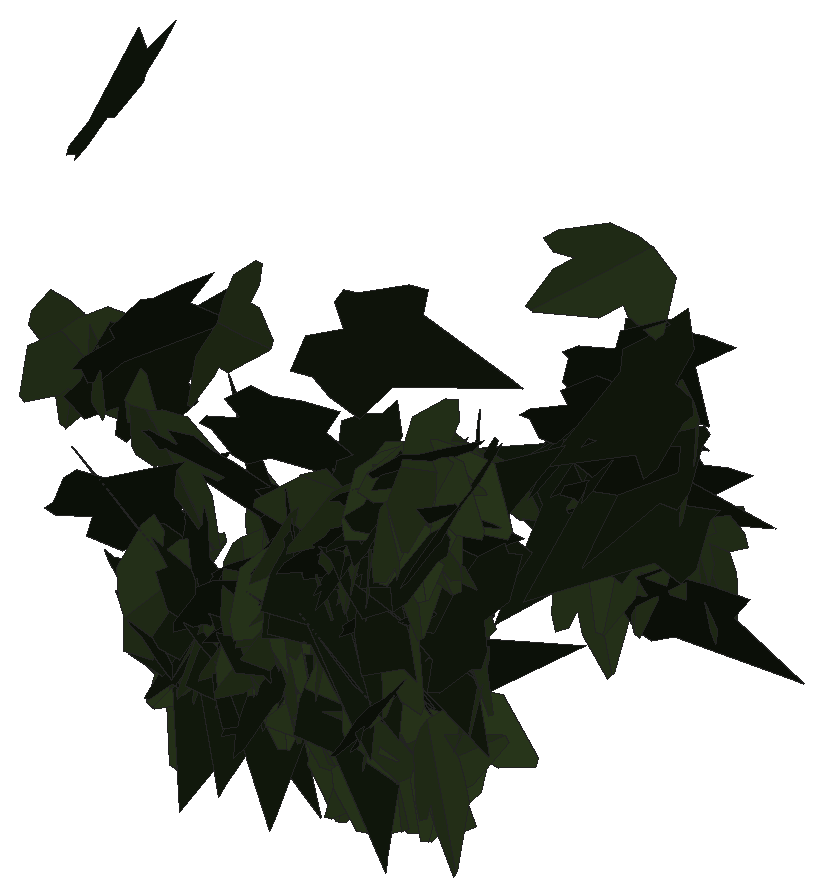
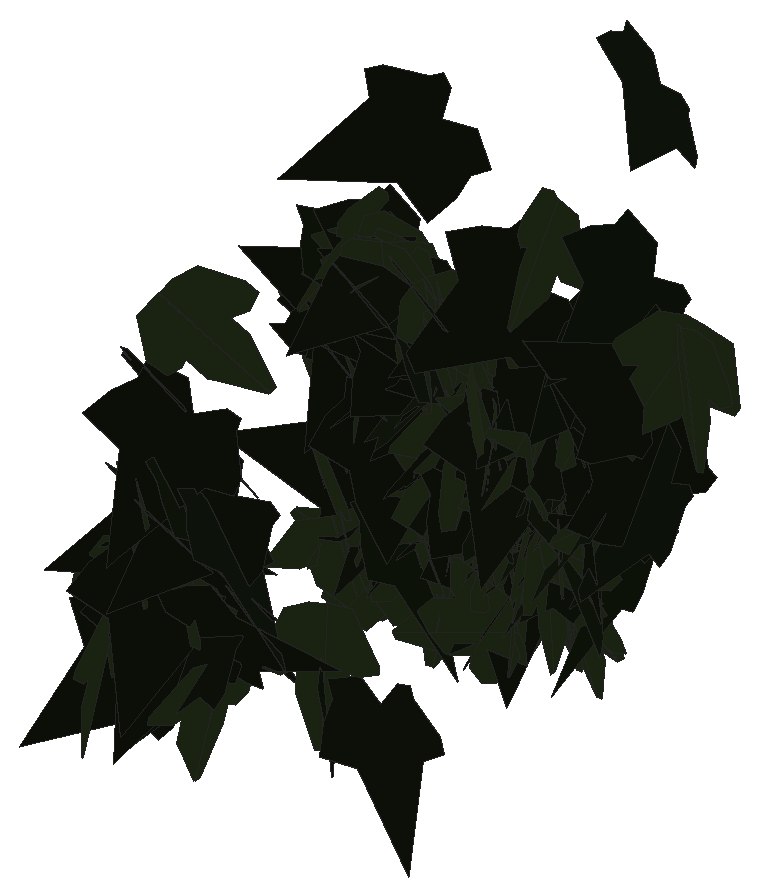
# SketchUp Ruby script. Lengths in inches.
U = 1.inch
M = Sketchup.active_model
def pt(a) = Geom::Point3d.new(a.map { |v| v * U })
def face(e, loops, mat)
  f = e.add_face(loops[0].map { |a| pt(a) })
  loops[1..].each { |l| e.add_face(l.map { |a| pt(a) }).erase! }
  f.material = f.back_material = mat if mat
  f
end
# faces: each face lists its corners as indices into pts; further lists are holes
def faces(e, pts, list, mat = nil) = list.each { |f| face(e, (f[0].is_a?(Array) ? f : [f]).map { |l| l.map { |i| pts[i] } }, mat) }
# xy, xz, yz: faces in a plane at the given z, y or x. An outline is a flat list of corners, or four numbers for a rectangle; further outlines are holes
def ring(l) = l.size == 4 ? [[l[0], l[1]], [l[2], l[1]], [l[2], l[3]], [l[0], l[3]]] : l.each_slice(2).to_a
def flat(e, list, mat, &to3) = list.each { |f| face(e, (f[0].is_a?(Array) ? f : [f]).map { |l| ring(l).map { |u, v| to3.(u, v) } }, mat) }
def xy(e, z, list, mat = nil) = flat(e, list, mat) { |x, y| [x, y, z] }
def xz(e, y, list, mat = nil) = flat(e, list, mat) { |x, z| [x, y, z] }
def yz(e, x, list, mat = nil) = flat(e, list, mat) { |y, z| [x, y, z] }
def lines(e, pts, list) = list.each { |a, b| e.add_line(pt(pts[a]), pt(pts[b])) }
# prism: a flat outline (further loops are holes) pulled along v
def prism(e, loops, v, mat = nil)
  f = face(e, loops, mat); d = Geom::Vector3d.new(v.map { |x| x * U })
  f.pushpull(f.normal.samedirection?(d) ? d.length : -d.length)
end
def box(e, o, s, mat = nil) = prism(e, [[o, [o[0] + s[0], o[1], o[2]], [o[0] + s[0], o[1] + s[1], o[2]], [o[0], o[1] + s[1], o[2]]]], [0, 0, s[2]], mat)
def at(x, y, z, deg = 0) = Geom::Transformation.translation(pt([x, y, z])) * Geom::Transformation.rotation(ORIGIN, Z_AXIS, deg.degrees)
def axes(o, x, y, z) = Geom::Transformation.new([*x, 0, *y, 0, *z, 0, *pt(o).to_a, 1])
def part(name) = M.definitions.add(name)
# library, detail: a bought-in or finely detailed component or shape, given as its bounding box
def library(name, o, s) = part(name).tap { |d| box(d.entities, o, s) }
def detail(e, o, s) = box(e.add_group.entities, o, s)
def put(e, d, t, mat = nil) = e.add_instance(d, t).tap { |i| i.material = mat if mat }
def group(e, t, mat = nil) = e.add_group.tap { |g| g.transformation = t; g.material = mat if mat }.entities
root = M.entities
M.materials.add("efeu1").color = [18, 25, 13]
M.materials.add("efeu2").color = [43, 57, 29]
c1 = part("ivyleaf_9")
p = [[1.54,2.16,1.25],[1.36,2.04,1.19],[-0.21,0.99,0.68],[-0.71,1.11,0.82],[-0.85,0.86,0.67],[-0.8,0.17,0.21],
  [-0.9,-0.01,0.1],[-0.67,-0.16,-0.02],[-0.08,-0.08,-0.05],[-0.03,-0.6,-0.4],[0.65,-0.88,-0.66],[0.83,-0.6,-0.49],
  [1.29,-0.42,-0.43],[1.8125,-0.07,-0.26],[1.21,0.44,0.15]]
faces(c1.entities,p,[[0,1,2,3,4,5,6,7,8,9,10,11,12,13,14]],"efeu1")
c2 = part("ivyleaf_10")
p = [[0,0.5,-0.03],[-0.0625,2.02,-0.43],[-0.19,2.01,-0.46],[-0.54,1.05,-0.29],[-0.52,0.625,-0.18],[-0.83,0.76,-0.28],
  [-1.16,0.64,-0.33],[-1.15,0.33,-0.24],[-0.77,-0.39,0.02],[-0.3,-0.51,0.16],[0.04,-0.48,0.23],[-0.02,2.01,-0.4375],
  [-0.06,2.01,-0.43],[0.04,-0.49,0.23],[0.67,-0.49,0.14],[1.38,0.36,-0.2],[1.375,0.51,-0.24],[0.81,0.65,-0.19],
  [0.62,0.59,-0.15],[0.6,1.09,-0.28],[0.5,1.23,-0.31]]
faces(c2.entities,p,[[0,1,2,3,4,5,6,7,8,9,10],[11,12,0,13,14,15,16,17,18,19,20]],"efeu2")
put(root,c1,axes([30.3,224.34,224.28],[0.36199,0.32235,-0.1227],[0.08167,0.09271,0.48449],[0.3351,-0.37081,0.01446]))
put(root,c2,axes([32.81,224.46,225.28],[-0.03829,-0.49672,-0.04244],[-0.01517,0.0437,-0.49786],[0.4983,-0.03683,-0.01841]))
put(root,c2,axes([30.12,224.32,225.76],[-0.34431,-0.24602,-0.26632],[0.22559,0.14214,-0.42297],[0.28383,-0.41142,0.01312]))
put(root,c1,axes([31.24,224.25,225.24],[0.49836,0.04008,-0.00536],[-0.00887,0.04369,-0.49801],[-0.03945,0.49647,0.04426]))
put(root,c1,axes([32.05,224.4,223.45],[-0.3806,0.32371,0.01877],[-0.01525,0.01104,-0.49965],[-0.3239,-0.3809,0.00148]))
put(root,c1,axes([31.45,224.68,223.42],[-0.37688,-0.29912,-0.13597],[0.14267,0.03742,-0.47775],[0.29598,-0.39891,0.05715]))
put(root,c2,axes([30.91,224.42,225.18],[-0.45546,0.1255,-0.16373],[0.1574,-0.0451,-0.47243],[-0.13335,-0.48189,0.00157]))
put(root,c2,axes([30,224.39,225.77],[0.44133,-0.1976,-0.12722],[-0.05473,0.17682,-0.46448],[0.22855,0.4239,0.13444]))
put(root,c2,axes([32.14,224.55,224.76],[0.14337,-0.47824,0.02696],[0.00611,-0.02632,-0.49927],[0.47896,0.14349,-0.0017]))
put(root,c2,axes([31.86,224.5625,223.79],[-0.30924,0.2654,-0.28972],[0.18417,-0.22777,-0.40522],[-0.34707,-0.35733,0.04311]))
put(root,c1,axes([32.98,224.1875,226.95],[0.03794,0.09374,-0.48967],[0.18461,0.45354,0.10112],[0.46312,-0.18846,-0.0002]))
put(root,c2,axes([33.05,224.51,224.05],[0.47753,-0.11742,-0.09043],[-0.08349,0.03892,-0.49144],[0.12245,0.48446,0.01756]))
put(root,c1,axes([33,224.52,225.51],[-0.45583,0.20506,-0.0131],[0.00986,-0.01002,-0.4998],[-0.20524,-0.45591,0.00509]))
put(root,c2,axes([31.29,224.49,223.57],[0.20122,-0.45427,-0.05611],[0.03844,0.07785,-0.4924],[0.4561,0.19385,0.06626]))
put(root,c2,axes([33.43,224.54,225.62],[0.4997,0.01296,-0.01164],[-0.01166,0.00038,-0.49986],[-0.01295,0.49983,0.00068]))
put(root,c1,axes([31.86,224.26,224.24],[0.16464,0.46751,-0.06579],[-0.01741,-0.06361,-0.49563],[-0.47179,0.16549,-0.00466]))
put(root,c2,axes([33.6,224.57,225.69],[0.3653,0.27747,-0.1989],[-0.17977,-0.09131,-0.45754],[-0.29024,0.4058,0.03305]))
put(root,c2,axes([33.35,224.46,225.56],[-0.44466,-0.17136,-0.15137],[0.16363,-0.00729,-0.47241],[0.1597,-0.46966,0.06256]))
put(root,c2,axes([32.6,224.5,225.06],[-0.44918,-0.20095,0.08865],[-0.0734,-0.05288,-0.49175],[0.20701,-0.45478,0.01801]))
put(root,c1,axes([30.7,224.1,226.14],[0.21613,0.35999,0.27146],[0.11023,0.24971,-0.41892],[-0.43719,0.24093,0.02858]))
put(root,c2,axes([33.17,224.45,225.08],[-0.49791,-0.04403,0.01222],[-0.0124,0.00159,-0.49984],[0.04398,-0.49805,-0.00267]))
put(root,c1,axes([30.5625,224.12,228.125],[0.0463,0.33401,0.36918],[-0.07892,0.37101,-0.32576],[-0.49156,-0.02811,0.08707]))
put(root,c1,axes([31.86,224.27,225.72],[0.45476,0.1337,0.15911],[0.153,0.04367,-0.47401],[-0.14065,0.47981,-0.00119]))
put(root,c1,axes([33.55,224.52,225.26],[-0.42667,0.25335,0.06137],[-0.07135,-0.00027,-0.49488],[-0.25072,-0.43106,0.03639]))
put(root,c2,axes([30.88,224.13,223.8],[0.02789,0.03793,-0.49778],[0.13057,0.48065,0.04394],[0.48184,-0.13244,0.0169]))
put(root,c2,axes([32.77,224.5,224.96],[0.31589,-0.354,-0.15778],[-0.09579,0.12593,-0.47431],[0.37555,0.32988,0.01174]))
put(root,c1,axes([32.53,224.69,224.5],[-0.01567,-0.49138,-0.09112],[-0.00161,0.09121,-0.49161],[0.49975,-0.01511,-0.00444]))
put(root,c1,axes([31.61,224.73,223.64],[-0.34414,-0.32276,-0.16552],[0.13104,0.10213,-0.47159],[0.33823,-0.36796,0.0143]))
put(root,c2,axes([33.3,224.49,225.59],[0.31849,0.37839,0.07338],[0.04371,0.05912,-0.49456],[-0.38296,0.32144,0.00458]))
put(root,c2,axes([31.68,224.52,224.18],[-0.04676,0.49437,-0.05844],[0.0001,-0.05868,-0.49654],[-0.49781,-0.04645,0.00539]))
put(root,c2,axes([32.6,224.48,224.96],[0.36442,-0.23007,-0.25351],[-0.18601,0.17777,-0.42872],[0.2874,0.40678,0.04398]))
put(root,c2,axes([33.35,224.51,225.26],[0.04972,0.49715,-0.01931],[-0.02432,-0.01696,-0.49912],[-0.49693,0.05057,0.02249]))
put(root,c2,axes([32.1,224.49,224.29],[0.25045,0.42741,0.06776],[0.03524,0.05789,-0.49539],[-0.43132,0.25291,-0.00112]))
put(root,c2,axes([31.39,224.61,223.27],[0.44892,-0.21518,-0.0466],[-0.04186,0.02049,-0.49782],[0.21615,0.45086,0.00038]))
put(root,c2,axes([31.78,224.46,223.94],[-0.34665,-0.25569,-0.25388],[0.24054,0.09808,-0.42722],[0.26828,-0.41833,0.05501]))
put(root,c1,axes([31.35,224.41,224.21],[0.10228,0.00438,-0.48941],[-0.48941,0.00532,-0.10223],[0.00431,0.49995,0.00537]))
put(root,c1,axes([31.7,224.8,223.33],[-0.02516,-0.4992,-0.0128],[0.00071,0.01278,-0.49984],[0.49937,-0.02516,0.00007]))
put(root,c1,axes([32.83,224.54,224.97],[-0.34487,0.35707,-0.05969],[0.03523,-0.04895,-0.49635],[-0.36031,-0.34656,0.0086]))
put(root,c2,axes([31.58,224.32,226.47],[-0.02562,-0.32422,-0.37977],[0.02402,0.37902,-0.32521],[0.49876,-0.03491,-0.00384]))
put(root,c1,axes([32.39,224.73,224.25],[0.09337,-0.48739,-0.0611],[-0.00082,0.06204,-0.49614],[0.4912,0.09275,0.01078]))
put(root,c1,axes([32.88,224.51,224.92],[-0.0032,0.44388,-0.23014],[-0.06967,-0.22829,-0.43935],[-0.49511,0.02925,0.06332]))
put(root,c1,axes([32.59,224.64,224.52],[-0.14359,-0.35991,-0.31598],[0.18205,0.2641,-0.38355],[0.44299,-0.2252,0.0552]))
put(root,c1,axes([32.6,224.78,223.25],[0.10058,-0.48957,0.01421],[0.00681,-0.01311,-0.49978],[0.48973,0.10073,0.00403]))
put(root,c1,axes([32.97,224.39,223.22],[0.05274,0.49685,0.01892],[-0.00193,-0.01882,0.49964],[0.49721,-0.05277,-0.00007]))
put(root,c1,axes([32.4,224.57,223.78],[0.43778,-0.23928,0.03305],[0.02907,-0.01573,-0.49891],[0.2398,0.43875,0.00014]))
put(root,c2,axes([32.85,224.89,222.76],[-0.17744,-0.18713,-0.42836],[-0.27686,-0.3271,0.25758],[-0.37664,0.32861,0.01246]))
put(root,c2,axes([32,224.6,223.6],[-0.09185,-0.48876,-0.05174],[0.00474,0.05176,-0.49729],[0.49147,-0.09185,-0.00488]))
put(root,c1,axes([30.59,224.38,223.61],[0.40946,-0.07041,-0.27819],[-0.24524,0.16583,-0.40294],[0.14901,0.46641,0.10126]))
put(root,c1,axes([33.86,224.43,225.54],[-0.22701,0.43879,0.07699],[-0.02501,0.07371,-0.4939],[-0.44479,-0.2281,-0.01152]))
put(root,c2,axes([31.67,224.67,223.65],[0.03199,-0.49883,-0.01207],[0.00001,0.0121,-0.49985],[0.49898,0.03198,0.00078]))
put(root,c1,axes([31.32,224.33,223.51],[-0.11731,0.40517,0.26847],[-0.11976,0.24357,-0.41992],[-0.47106,-0.16282,0.0399]))
put(root,c1,axes([30.17,224.51,224.46],[0.47288,-0.11244,-0.11724],[-0.10971,0.04507,-0.48573],[0.1198,0.4851,0.01796]))
put(root,c1,axes([31.51,224.65,223.65],[0.34569,-0.3611,-0.01008],[0.05427,0.06571,-0.49268],[0.35714,0.33954,0.08462]))
put(root,c2,axes([32.14,224.6,224.41],[-0.36525,0.33105,-0.08364],[0.05588,-0.06287,-0.49287],[-0.33685,-0.36939,0.00893]))
put(root,c2,axes([31.04,224.7,223.12],[0.47205,-0.16472,-0.00586],[-0.0047,0.00431,-0.49996],[0.16476,0.47207,0.00252]))
put(root,c1,axes([31.02,224.375,224.01],[0.38554,-0.03908,-0.31596],[-0.26335,0.23969,-0.35099],[0.1789,0.43706,0.16424]))
put(root,c2,axes([31.88,224.61,223.6875],[0.23827,0.43931,0.01538],[0.00833,0.01297,-0.49976],[-0.4395,0.23841,-0.00114]))
put(root,c1,axes([32.04,224.625,223.93],[-0.06961,0.42991,-0.24563],[-0.07281,-0.25424,-0.42434],[-0.48975,-0.02331,0.098]))
put(root,c2,axes([32.125,224.7,224.03],[-0.05275,-0.49721,-0.00051],[-0.0003,0.00054,-0.5],[0.49721,-0.05275,-0.00035]))
put(root,c2,axes([33.51,224.625,223.12],[-0.09083,0.49094,-0.02695],[0.00194,-0.02705,-0.49926],[-0.49168,-0.0908,0.00301]))
put(root,c2,axes([32.33,224.51,224.02],[0.27172,-0.20687,-0.3652],[-0.23163,0.2889,-0.33599],[0.35002,0.35177,0.06116]))
put(root,c2,axes([32.45,224.66,224.61],[-0.48803,0.09488,0.05317],[-0.06693,-0.0693,-0.49063],[-0.08573,-0.486,0.08034]))
put(root,c2,axes([33.5,224.38,225.82],[0.01346,-0.24934,-0.43319],[0.16225,0.41206,-0.23213],[0.47275,-0.13432,0.09201]))
put(root,c2,axes([32.57,224.78,223.12],[-0.35216,-0.34422,0.08658],[0.01571,-0.13696,-0.48062],[0.3546,-0.33579,0.10727]))
put(root,c1,axes([34.01,224.54,224.55],[-0.29796,0.27833,0.28941],[-0.21545,0.19329,-0.4077],[-0.33883,-0.36766,0.00475]))
put(root,c1,axes([33.15,224.7,224.42],[0.1747,-0.42786,-0.19084],[-0.00516,0.20191,-0.45739],[0.46846,0.16178,0.06613]))
put(root,c1,axes([33.375,224.44,225.06],[0.00619,0.00028,0.49996],[0.4729,0.16226,-0.00594],[-0.16225,0.47294,0.00175]))
put(root,c1,axes([33.19,224.3125,225.61],[0.32859,0.3029,0.22423],[0.09206,0.22398,-0.43745],[-0.36545,0.32877,0.09143]))
put(root,c2,axes([31.24,224.77,223.4],[0.42305,-0.0053,-0.26645],[-0.2665,-0.0045,-0.42304],[0.00209,0.49995,-0.00663]))
put(root,c1,axes([33.35,224.46,225.15],[0.37723,0.32662,-0.0319],[-0.01898,-0.02682,-0.49892],[-0.32763,0.37762,-0.00784]))
put(root,c2,axes([32.41,224.65,223.02],[-0.49881,0.03189,-0.01316],[0.01301,-0.00282,-0.49982],[-0.03195,-0.49897,0.00199]))
put(root,c2,axes([32.8,224.63,224.86],[0.31205,-0.36083,-0.14976],[0.015,0.20259,-0.45687],[0.39039,0.28064,0.13726]))
put(root,c1,axes([31.48,224.74,223.28],[0.27046,-0.39556,-0.14278],[-0.08257,0.1165,-0.47918],[0.41235,0.28277,-0.0023]))
put(root,c1,axes([31.92,224.6,224.4],[0.09363,-0.17736,0.45801],[-0.1806,0.42116,0.20001],[-0.45674,-0.20289,0.01481]))
put(root,c1,axes([31.25,224.55,223.58],[0.49811,0.04244,-0.00934],[-0.01129,0.02258,-0.49936],[-0.04196,0.49768,0.02345]))
put(root,c1,axes([31.83,224.64,223.93],[0.44406,-0.2255,0.04427],[0.10052,0.10399,-0.47863],[0.20665,0.43398,0.13769]))
put(root,c2,axes([32.34,224.62,224.43],[0.13376,0.47382,0.08717],[-0.0554,0.10499,-0.4857],[-0.47858,0.12028,0.08058]))
put(root,c2,axes([32.66,224.77,223.54],[0.23852,0.43288,-0.07566],[-0.04254,-0.06294,-0.4942],[-0.43738,0.24219,0.00681]))
put(root,c1,axes([32.67,224.69,224.67],[0.37045,-0.32576,-0.08156],[0.02413,0.14694,-0.47731],[0.33494,0.3497,0.12459]))
put(root,c2,axes([31.26,224.75,223.48],[0.0405,-0.49155,-0.0821],[0.01724,0.0837,-0.49264],[0.49806,0.03707,0.02373]))
put(root,c2,axes([31.53,224.77,223.35],[-0.18545,-0.45836,-0.07426],[0.04571,0.06156,-0.49409],[0.46208,-0.19005,0.01907]))
put(root,c1,axes([31.83,224.49,224.38],[0.14163,0.47564,0.06085],[-0.0301,0.07214,-0.49385],[-0.47857,0.13623,0.04907]))
put(root,c2,axes([32.14,224.6,224.06],[-0.33084,0.26799,0.26216],[-0.2152,0.15054,-0.42547],[-0.30698,-0.39436,0.01573]))
put(root,c2,axes([31.84,224.67,224.06],[0.41877,0.01933,0.2725],[-0.27118,0.08965,0.41039],[-0.033,-0.49152,0.08557]))
put(root,c2,axes([33.01,224.69,222.49],[0.06564,0.48943,-0.07844],[0.01477,0.07716,0.49379],[0.49545,-0.06714,-0.00433]))
put(root,c2,axes([32.61,224.87,223.21],[0.3514,-0.35349,-0.03959],[-0.02626,0.02972,-0.49842],[0.35472,0.35237,0.00232]))
put(root,c2,axes([33.07,224.6875,222.62],[-0.22767,-0.19052,0.40233],[0.30842,0.25836,0.29687],[-0.32101,0.38335,-0.00012]))
put(root,c1,axes([31.68,224.68,223.49],[0.29649,0.33224,-0.2274],[-0.15624,-0.16532,-0.44526],[-0.37106,0.33509,0.00578]))
put(root,c1,axes([32.78,224.7,223.9],[0.46611,-0.06571,-0.16859],[-0.1659,0.03078,-0.47067],[0.07223,0.49471,0.00689]))
put(root,c1,axes([33.64,224.8,224.61],[-0.08544,0.16725,0.46339],[-0.4582,0.14579,-0.1371],[-0.18098,-0.44808,0.12835]))
put(root,c2,axes([33.46,224.9,224.45],[-0.365,0.24836,-0.23471],[0.17146,-0.16396,-0.44013],[-0.29559,-0.40179,0.03452]))
put(root,c1,axes([30.34,224.59,225.22],[0.02384,-0.08024,0.49294],[0.40385,0.29344,0.02824],[-0.29383,0.3968,0.0788]))
put(root,c2,axes([32.14,224.74,224.03],[-0.33133,-0.15695,-0.33998],[0.3158,0.12684,-0.36631],[0.20123,-0.45747,0.01508]))
put(root,c2,axes([31.45,224.77,223.4],[0.11264,-0.41577,-0.25387],[0.02633,0.26539,-0.42294],[0.48643,0.08191,0.08169]))
put(root,c2,axes([32.42,224.76,222.84],[-0.19357,0.42045,-0.18908],[-0.07828,0.17212,0.46287],[0.45431,0.2088,-0.00081]))
put(root,c1,axes([33.125,224.73,223.62],[0.19554,-0.01627,0.45989],[0.45371,0.09032,-0.18972],[-0.0769,0.49151,0.05009]))
put(root,c1,axes([32.96,224.72,224.18],[0.1045,0.48876,0.01386],[0.00471,0.01316,-0.4998],[-0.48893,0.10459,-0.00185]))
put(root,c2,axes([33.54,225.05,223.77],[0.35875,-0.34611,-0.03888],[-0.02917,0.02577,-0.49848],[0.34706,0.35993,-0.00171]))
put(root,c2,axes([33.33,225.09,223.15],[0.36153,0.33032,-0.1009],[-0.07064,-0.07225,-0.48968],[-0.33809,0.36833,-0.00557]))
put(root,c1,axes([32.8,225,223.37],[-0.27068,0.41811,-0.04372],[0.02264,-0.03742,-0.49808],[-0.41978,-0.27163,0.00133]))
put(root,c2,axes([31.55,225.15,222.83],[0.10962,0.0631,0.48374],[0.44106,0.19903,-0.12592],[-0.20845,0.45432,-0.01202]))
put(root,c1,axes([33.84,227.16,225.46],[-0.46496,0.17506,0.05627],[-0.0528,0.01946,-0.49682],[-0.17614,-0.46795,0.00039]))
put(root,c2,axes([33.29,227.29,226.33],[0.26675,0.18935,-0.37814],[-0.40973,0.00499,-0.28653],[-0.10473,0.46273,0.15782]))
put(root,c1,axes([33.43,227.65,224.16],[-0.4085,-0.24006,0.15969],[-0.10114,-0.14002,-0.46922],[0.27,-0.41565,0.06584]))
put(root,c1,axes([32.86,227.62,223.95],[-0.49686,-0.03736,-0.04162],[0.0411,0.00839,-0.49824],[0.03792,-0.49853,-0.00526]))
put(root,c1,axes([33.1,227.23,224.3125],[0.40259,0.10625,0.27683],[0.26907,0.06523,-0.41635],[-0.12459,0.48421,-0.00465]))
put(root,c1,axes([33.4375,227.71,224.61],[-0.46481,-0.00097,-0.18427],[0.17685,-0.14285,-0.44533],[-0.05178,-0.47916,0.13313]))
put(root,c1,axes([31.72,227.24,222.95],[0.01915,-0.0198,0.49924],[-0.03743,0.49815,0.0212],[-0.49823,-0.03818,0.0176]))
put(root,c2,axes([33.01,227.59,223.76],[0.49086,-0.09454,-0.01095],[-0.00454,0.03417,-0.49881],[0.09506,0.48979,0.03269]))
put(root,c1,axes([33.15,227.51,224.77],[-0.34486,0.36087,-0.02903],[0.0191,-0.0219,-0.49915],[-0.36153,-0.34539,0.00132]))
put(root,c2,axes([31.6,227.5,223.81],[-0.48919,-0.00928,0.10298],[-0.10307,0.00413,-0.48924],[0.00823,-0.4999,-0.00596]))
put(root,c2,axes([33.1875,227.56,224.01],[-0.48082,-0.11722,-0.07122],[0.06888,0.01813,-0.4949],[0.1186,-0.48573,-0.00129]))
put(root,c1,axes([32.69,227.53,224.57],[-0.26649,0.42137,0.03789],[-0.03353,0.02361,-0.49832],[-0.42174,-0.26813,0.01568]))
put(root,c2,axes([33.18,227.67,223.72],[-0.45579,0.19245,0.07225],[-0.1097,-0.0791,-0.48136],[-0.17385,-0.45465,0.11433]))
put(root,c1,axes([30.92,227.52,223.29],[-0.09843,0.48883,-0.03683],[0.00841,-0.03587,-0.49864],[-0.49014,-0.09879,-0.00116]))
put(root,c1,axes([33.11,227.45,225.39],[0.35234,0.35474,0.00439],[0.00729,-0.00105,-0.49995],[-0.35469,0.35236,-0.00591]))
put(root,c1,axes([32.66,227.43,224.74],[0.39004,0.27891,0.14168],[0.09189,0.11432,-0.478],[-0.29904,0.39892,0.03792]))
put(root,c2,axes([33.4,227.75,223.94],[-0.49246,-0.08314,-0.02397],[0.02206,0.01332,-0.49934],[0.08367,-0.49286,-0.00945]))
put(root,c1,axes([32.65,227.84,223.61],[-0.25043,0.13509,0.41114],[-0.39378,0.12589,-0.28122],[-0.1795,-0.46465,0.04334]))
put(root,c2,axes([33.54,227.75,224.66],[0.29453,-0.31079,-0.25819],[-0.13344,0.22676,-0.42518],[0.38137,0.31936,0.05063]))
put(root,c1,axes([33.31,227.65,223.11],[0.46681,0.12893,0.12435],[0.1207,0.03007,-0.48428],[-0.13235,0.48216,-0.00305]))
put(root,c2,axes([32.54,227.8,223.14],[0.05963,0.49401,0.04894],[-0.02268,0.05196,-0.49678],[-0.49591,0.05703,0.02861]))
put(root,c1,axes([32.57,227.78,223.64],[0.48092,-0.07297,-0.11573],[-0.11249,0.02982,-0.48627],[0.07787,0.49375,0.01227]))
put(root,c1,axes([32.92,227.73,223.68],[0.37504,0.32593,-0.05579],[-0.04302,-0.03554,-0.49688],[-0.32786,0.3775,0.00138]))
put(root,c1,axes([33.09,227.75,223.96],[0.22685,0.44542,-0.01175],[-0.01149,-0.00733,-0.49981],[-0.44543,0.22704,0.00691]))
put(root,c2,axes([33.5,228.13,223.34],[-0.19527,0.4156,0.19785],[-0.13424,0.15416,-0.45631],[-0.44028,-0.23133,0.05137]))
